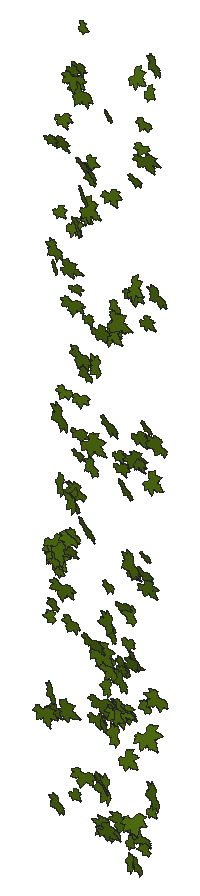
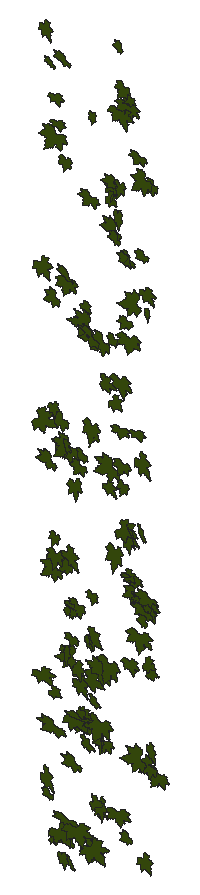
# SketchUp Ruby script. Lengths in inches.
U = 1.inch
M = Sketchup.active_model
def pt(a) = Geom::Point3d.new(a.map { |v| v * U })
def face(e, loops, mat)
  f = e.add_face(loops[0].map { |a| pt(a) })
  loops[1..].each { |l| e.add_face(l.map { |a| pt(a) }).erase! }
  f.material = f.back_material = mat if mat
  f
end
# faces: each face lists its corners as indices into pts; further lists are holes
def faces(e, pts, list, mat = nil) = list.each { |f| face(e, (f[0].is_a?(Array) ? f : [f]).map { |l| l.map { |i| pts[i] } }, mat) }
# xy, xz, yz: faces in a plane at the given z, y or x. An outline is a flat list of corners, or four numbers for a rectangle; further outlines are holes
def ring(l) = l.size == 4 ? [[l[0], l[1]], [l[2], l[1]], [l[2], l[3]], [l[0], l[3]]] : l.each_slice(2).to_a
def flat(e, list, mat, &to3) = list.each { |f| face(e, (f[0].is_a?(Array) ? f : [f]).map { |l| ring(l).map { |u, v| to3.(u, v) } }, mat) }
def xy(e, z, list, mat = nil) = flat(e, list, mat) { |x, y| [x, y, z] }
def xz(e, y, list, mat = nil) = flat(e, list, mat) { |x, z| [x, y, z] }
def yz(e, x, list, mat = nil) = flat(e, list, mat) { |y, z| [x, y, z] }
def lines(e, pts, list) = list.each { |a, b| e.add_line(pt(pts[a]), pt(pts[b])) }
# prism: a flat outline (further loops are holes) pulled along v
def prism(e, loops, v, mat = nil)
  f = face(e, loops, mat); d = Geom::Vector3d.new(v.map { |x| x * U })
  f.pushpull(f.normal.samedirection?(d) ? d.length : -d.length)
end
def box(e, o, s, mat = nil) = prism(e, [[o, [o[0] + s[0], o[1], o[2]], [o[0] + s[0], o[1] + s[1], o[2]], [o[0], o[1] + s[1], o[2]]]], [0, 0, s[2]], mat)
def at(x, y, z, deg = 0) = Geom::Transformation.translation(pt([x, y, z])) * Geom::Transformation.rotation(ORIGIN, Z_AXIS, deg.degrees)
def axes(o, x, y, z) = Geom::Transformation.new([*x, 0, *y, 0, *z, 0, *pt(o).to_a, 1])
def part(name) = M.definitions.add(name)
# library, detail: a bought-in or finely detailed component or shape, given as its bounding box
def library(name, o, s) = part(name).tap { |d| box(d.entities, o, s) }
def detail(e, o, s) = box(e.add_group.entities, o, s)
def put(e, d, t, mat = nil) = e.add_instance(d, t).tap { |i| i.material = mat if mat }
def group(e, t, mat = nil) = e.add_group.tap { |g| g.transformation = t; g.material = mat if mat }.entities
root = M.entities
M.materials.add("[Vegetation Blur 03]").color = [83, 114, 18]
c1 = part("ivy")
xy(c1.entities,0,[[0.782,0,0.786,0,0.787,0.005,0.789,0.009,0.821,0.072,0.875,0.147,1.001,0.272,1.073,0.331,1.137,0.363,1.178,0.379,1.223,0.384,1.272,0.383,1.311,0.374,1.36,0.355,1.399,0.334,1.491,0.285,1.541,0.244,1.583,0.199,1.617,0.15,1.64,0.128,1.662,0.115,1.717,0.105,1.745,0.093,1.784,0.054,1.819,0.057,1.854,0.064,1.882,0.075,1.896,0.074,1.91,0.071,1.937,0.063,1.964,0.053,1.99,0.038,2.016,0.015,2.034,0.002,2.04,0,2.038,0.003,2.036,0.007,2.033,0.038,2.036,0.068,2.045,0.1,2.055,0.116,2.064,0.123,2.077,0.129,2.088,0.129,2.106,0.132,2.118,0.13,2.179,0.132,2.207,0.133,2.225,0.133,2.242,0.138,2.22,0.162,2.207,0.186,2.206,0.213,2.212,0.236,2.228,0.262,2.247,0.274,2.298,0.283,2.355,0.294,2.37,0.296,2.376,0.295,2.377,0.3,2.377,0.303,2.385,0.329,2.411,0.37,2.426,0.392,2.449,0.407,2.511,0.426,2.561,0.444,2.619,0.466,2.589,0.469,2.561,0.476,2.501,0.5,2.449,0.516,2.424,0.523,2.401,0.535,2.377,0.556,2.372,0.568,2.36,0.575,2.268,0.586,2.225,0.592,2.207,0.599,2.194,0.61,2.143,0.65,2.13,0.664,2.122,0.682,2.123,0.7,2.13,0.719,2.148,0.75,2.17,0.781,2.195,0.807,2.221,0.828,2.284,0.874,2.291,0.88,2.288,0.887,2.276,0.9,2.267,0.916,2.265,0.933,2.273,0.967,2.292,1.002,2.313,1.03,2.334,1.054,2.348,1.067,2.358,1.074,2.363,1.076,2.362,1.081,2.35,1.094,2.347,1.11,2.35,1.143,2.359,1.18,2.385,1.254,2.415,1.324,2.448,1.393,2.45,1.4,2.446,1.398,2.44,1.394,2.427,1.383,2.402,1.36,2.376,1.339,2.345,1.324,2.305,1.309,2.282,1.303,2.273,1.306,2.245,1.294,2.212,1.287,2.187,1.291,2.163,1.301,2.142,1.316,2.134,1.327,2.124,1.325,2.09,1.292,2.053,1.259,2.014,1.234,1.973,1.215,1.954,1.21,1.931,1.208,1.909,1.212,1.893,1.22,1.879,1.233,1.872,1.248,1.867,1.281,1.864,1.319,1.821,1.258,1.773,1.197,1.726,1.141,1.698,1.121,1.679,1.116,1.666,1.117,1.647,1.122,1.632,1.129,1.62,1.141,1.617,1.154,1.617,1.219,1.621,1.254,1.623,1.268,1.623,1.281,1.618,1.314,1.606,1.346,1.603,1.375,1.607,1.403,1.603,1.467,1.599,1.499,1.605,1.525,1.614,1.552,1.629,1.577,1.635,1.589,1.629,1.587,1.618,1.582,1.596,1.566,1.581,1.556,1.568,1.552,1.557,1.55,1.545,1.553,1.531,1.562,1.522,1.572,1.504,1.591,1.486,1.611,1.474,1.631,1.457,1.666,1.455,1.684,1.457,1.698,1.452,1.715,1.444,1.728,1.424,1.754,1.419,1.772,1.423,1.786,1.434,1.819,1.444,1.848,1.446,1.855,1.44,1.861,1.43,1.867,1.386,1.904,1.349,1.948,1.326,1.973,1.31,1.995,1.288,2.048,1.284,2.153,1.287,2.254,1.284,2.255,1.282,2.253,1.278,2.247,1.274,2.237,1.266,2.216,1.226,2.125,1.208,2.076,1.184,2.033,1.155,1.984,1.135,1.942,1.111,1.899,1.083,1.861,1.053,1.85,1.059,1.83,1.061,1.809,1.056,1.79,1.049,1.767,1.04,1.749,1.018,1.733,0.994,1.726,0.942,1.734,0.95,1.6875,0.944,1.645,0.932,1.608,0.911,1.585,0.881,1.58,0.854,1.582,0.828,1.588,0.785,1.618,0.773,1.625,0.775,1.614,0.779,1.598,0.796,1.502,0.818,1.402,0.861,1.283,0.882,1.224,0.894,1.174,0.892,1.148,0.886,1.123,0.881,1.107,0.872,1.099,0.849,1.094,0.818,1.092,0.789,1.098,0.762,1.107,0.753,1.113,0.721,1.139,0.698,1.163,0.678,1.194,0.665,1.224,0.628,1.28,0.612,1.312,0.606,1.327,0.606,1.314,0.599,1.282,0.594,1.267,0.581,1.256,0.544,1.245,0.512,1.244,0.473,1.249,0.444,1.256,0.382,1.288,0.339,1.306,0.324,1.316,0.317,1.324,0.309,1.326,0.27,1.314,0.227,1.313,0.185,1.3125,0.152,1.317,0.122,1.328,0.092,1.345,0.073,1.353,0.079,1.338,0.092,1.308,0.117,1.249,0.13,1.215,0.139,1.164,0.147,1.148,0.157,1.136,0.163,1.122,0.174,1.086,0.177,1.067,0.182,1.054,0.186,1.043,0.191,1.038,0.211,1.028,0.237,1.005,0.25,0.974,0.253,0.96,0.25,0.944,0.242,0.914,0.243,0.906,0.249,0.902,0.26,0.894,0.289,0.88,0.307,0.873,0.322,0.862,0.364,0.799,0.403,0.738,0.431,0.709,0.439,0.691,0.441,0.678,0.4375,0.66,0.428,0.645,0.394,0.623,0.303,0.594,0.255,0.581,0.214,0.577,0.179,0.573,0.173,0.568,0.175,0.561,0.167,0.55,0.141,0.523,0.113,0.503,0.077,0.49,0.045,0.486,0.026,0.485,0.019,0.486,0.011,0.483,0,0.471,0.014,0.467,0.044,0.455,0.058,0.447,0.07,0.438,0.097,0.411,0.125,0.394,0.158,0.377,0.174,0.366,0.182,0.359,0.185,0.361,0.242,0.331,0.253,0.316,0.258,0.303,0.262,0.283,0.274,0.278,0.308,0.274,0.341,0.252,0.366,0.226,0.366,0.222,0.37,0.22,0.38,0.221,0.395,0.221,0.425,0.216,0.45,0.207,0.465,0.192,0.473,0.178,0.484,0.15,0.489,0.116,0.483,0.089,0.468,0.058,0.45,0.035,0.435,0.018,0.429,0.011,0.434,0.012,0.438,0.014,0.469,0.019,0.542,0.016,0.581,0.015,0.612,0.027,0.68,0.055,0.696,0.057,0.712,0.052,0.73,0.045,0.741,0.036,0.766,0.014]])
put(root,c1,axes([19.03,173.2,108.03],[0.55674,-0.05035,0.19483],[0.23814,-0.03752,-0.45478],[-0.02967,-1.24598,0.00582]),"[Vegetation Blur 03]")
put(root,c1,axes([20.39,173.2,113.54],[0.04662,-0.02211,-0.24119],[-0.29524,-0.03871,-0.03745],[0.01692,-0.61444,0.01104]),"[Vegetation Blur 03]")
put(root,c1,axes([20.4,173.2,114.15],[0.07372,0.06524,-0.26494],[-0.3259,0.04312,-0.05873],[-0.01352,-0.68368,-0.02899]),"[Vegetation Blur 03]")
put(root,c1,axes([20.1,173.2,109.72],[0.32192,-0.21102,-0.29136],[-0.33943,0.22769,-0.27574],[-0.15085,-0.96265,-0.00135]),"[Vegetation Blur 03]")
put(root,c1,axes([20.15,173.2,116.78],[0.30881,-0.07275,-0.21101],[-0.25864,0.02403,-0.25343],[-0.03462,-0.82843,0.01118]),"[Vegetation Blur 03]")
put(root,c1,axes([19.68,173.2,138.69],[0.29342,-0.08692,0.17033],[0.21238,0.06683,-0.23833],[-0.01533,-0.73794,-0.04165]),"[Vegetation Blur 03]")
put(root,c1,axes([20.23,173.2,133.52],[0.38178,-0.11889,-0.25625],[-0.31299,0.05919,-0.31491],[-0.06294,-1.01546,0.01165]),"[Vegetation Blur 03]")
put(root,c1,axes([20.39,173.2,103.86],[0.3336,-0.07994,-0.30777],[-0.37102,0.14358,-0.27372],[-0.07791,-1.02608,-0.01433]),"[Vegetation Blur 03]")
put(root,c1,axes([20.31,173.2,132.32],[0.23472,-0.16453,-0.13977],[-0.15775,0.13898,-0.20218],[-0.10411,-0.58153,-0.00877]),"[Vegetation Blur 03]")
put(root,c1,axes([19.62,173.2,117.02],[0.386,0.08915,0.27036],[0.33331,-0.03157,-0.31533],[0.02283,-1.04625,0.03255]),"[Vegetation Blur 03]")
put(root,c1,axes([19.72,173.2,108.09],[0.30498,-0.11066,0.28031],[0.34736,0.05892,-0.24807],[-0.01408,-0.94337,-0.04838]),"[Vegetation Blur 03]")
put(root,c1,axes([20.63,173.2,124.82],[0.38094,-0.16652,-0.42659],[-0.51102,0.22607,-0.31784],[-0.13644,-1.3116,-0.00062]),"[Vegetation Blur 03]")
put(root,c1,axes([20.95,173.2,120.95],[0.09708,-0.16375,-0.35064],[-0.41312,0.26056,-0.09533],[-0.14231,-0.86813,0.03753]),"[Vegetation Blur 03]")
put(root,c1,axes([19.56,173.2,116.8125],[0.58138,0.04851,0.24502],[0.30111,-0.07156,-0.47365],[0.00495,-1.34457,0.03405]),"[Vegetation Blur 03]")
put(root,c1,axes([20.21,173.2,134.86],[0.2013,0.04338,0.20783],[0.25534,-0.0094,-0.16443],[0.00948,-0.6679,0.01581]),"[Vegetation Blur 03]")
put(root,c1,axes([19.92,173.2,116.17],[0.3314,0.11464,0.31783],[0.39311,-0.13672,-0.26526],[-0.0151,-1.04335,0.06968]),"[Vegetation Blur 03]")
put(root,c1,axes([20.36,173.2,115.56],[0.07858,-0.01385,0.24493],[0.29907,-0.05144,-0.06436],[-0.02588,-0.6363,-0.00013]),"[Vegetation Blur 03]")
put(root,c1,axes([20.08,173.2,115.3],[0.62015,-0.02976,-0.03519],[-0.04222,0.07375,-0.50547],[-0.01689,-1.27709,-0.02837]),"[Vegetation Blur 03]")
put(root,c1,axes([19.98,173.2,138.72],[0.41952,-0.13561,0.24997],[0.31292,0.12999,-0.33871],[-0.01528,-1.06095,-0.07345]),"[Vegetation Blur 03]")
put(root,c1,axes([20.68,173.2,125.82],[0.33208,0.00162,-0.09351],[-0.114,-0.06757,-0.26985],[0.01145,-0.71971,0.02513]),"[Vegetation Blur 03]")
put(root,c1,axes([20.31,173.2,140.02],[0.3458,0.03513,0.16386],[0.2014,-0.03386,-0.28195],[0.00648,-0.82214,0.01861]),"[Vegetation Blur 03]")
put(root,c1,axes([21.78,173.2,120.7],[0.10352,-0.20906,-0.49577],[-0.59692,0.27823,-0.10147],[-0.15173,-1.23717,0.06096]),"[Vegetation Blur 03]")
put(root,c1,axes([20.39,173.2,108.02],[0.20638,-0.06433,0.46905],[0.57546,0.04752,-0.16762],[0.01121,-1.25569,-0.03037]),"[Vegetation Blur 03]")
put(root,c1,axes([20.77,173.2,118.04],[0.4452,0.01529,-0.01974],[-0.02317,-0.10578,-0.36101],[0.01016,-0.91136,0.04157]),"[Vegetation Blur 03]")
put(root,c1,axes([21.01,173.2,113.6875],[0.43906,-0.08807,-0.12908],[-0.15747,0.03053,-0.36003],[-0.0453,-0.95985,0.00039]),"[Vegetation Blur 03]")
put(root,c1,axes([20.74,173.2,130.61],[0.54749,0.01991,-0.01395],[-0.01748,0.04635,-0.4465],[0.00896,-1.12621,-0.01862]),"[Vegetation Blur 03]")
put(root,c1,axes([21.77,173.2,120.92],[0.16632,0.09986,-0.39596],[-0.48659,-0.03313,-0.13745],[0.03103,-1.05488,-0.03317]),"[Vegetation Blur 03]")
put(root,c1,axes([21.45,173.2,118.375],[0.23314,-0.02071,-0.23083],[-0.28282,0.0106,-0.19042],[-0.01038,-0.7542,0.00366]),"[Vegetation Blur 03]")
put(root,c1,axes([21.27,173.2,120.26],[0.37136,-0.15214,-0.22354],[-0.25515,0.22677,-0.30661],[-0.12403,-0.92207,-0.03852]),"[Vegetation Blur 03]")
put(root,c1,axes([20.87,173.2,116.9],[0.22705,-0.08947,0.23456],[0.29067,0.06726,-0.18337],[-0.00101,-0.75069,-0.04439]),"[Vegetation Blur 03]")
put(root,c1,axes([20.73,173.2,131.78],[0.15315,-0.11376,0.42127],[0.51825,0.09795,-0.12133],[0.03021,-1.10363,-0.05419]),"[Vegetation Blur 03]")
put(root,c1,axes([21.71,173.2,135.02],[0.17953,-0.09504,-0.30608],[-0.36446,0.18198,-0.15128],[-0.09974,-0.83603,0.00186]),"[Vegetation Blur 03]")
put(root,c1,axes([20.84,173.2,142.68],[0.55862,-0.01173,0.01902],[0.02312,-0.03492,-0.45573],[-0.0064,-1.15001,0.01364]),"[Vegetation Blur 03]")
put(root,c1,axes([21.03,173.2,142.86],[0.27413,-0.06194,0.16545],[0.20434,0.02916,-0.2238],[-0.01572,-0.70099,-0.02393]),"[Vegetation Blur 03]")
put(root,c1,axes([21.14,173.2,131.2],[0.28384,0.00263,0.11756],[0.14245,0.09199,-0.22943],[0.02136,-0.64851,-0.03207]),"[Vegetation Blur 03]")
put(root,c1,axes([20.98,173.2,134.24],[0.23996,0.10055,0.29847],[0.36879,-0.09254,-0.19259],[-0.01117,-0.89532,0.05342]),"[Vegetation Blur 03]")
put(root,c1,axes([21.18,173.2,104.02],[0.1988,-0.0106,0.20658],[0.25313,-0.00387,-0.16228],[-0.00466,-0.6623,-0.00236]),"[Vegetation Blur 03]")
put(root,c1,axes([21.41,173.2,122.61],[0.33381,-0.09287,0.01816],[0.028,0.08748,-0.27236],[-0.04181,-0.68286,-0.03736]),"[Vegetation Blur 03]")
put(root,c1,axes([21.28,173.2,123.66],[0.39754,-0.01789,0.09307],[0.11433,0.03939,-0.32408],[-0.00307,-0.85015,-0.01697]),"[Vegetation Blur 03]")
put(root,c1,axes([21.41,173.2,125.57],[0.37993,0.04432,0.03279],[0.04106,-0.03097,-0.31026],[0.01982,-0.78558,0.01408]),"[Vegetation Blur 03]")
put(root,c1,axes([21.32,173.2,143.3125],[0.38821,-0.11193,0.10755],[0.13579,0.05066,-0.31818],[-0.04343,-0.84212,-0.03344]),"[Vegetation Blur 03]")
put(root,c1,axes([21.48,173.2,142.46],[0.60025,-0.11632,-0.20653],[-0.25299,0.02521,-0.49198],[-0.05685,-1.34025,0.00867]),"[Vegetation Blur 03]")
put(root,c1,axes([21.42,173.2,128.3],[0.58763,-0.14391,-0.14762],[-0.17735,0.08172,-0.48275],[-0.07846,-1.26257,-0.01442]),"[Vegetation Blur 03]")
put(root,c1,axes([21.45,173.2,105.64],[0.52025,0.05923,-0.06815],[-0.08303,-0.02209,-0.42521],[0.03012,-1.08405,0.00494]),"[Vegetation Blur 03]")
put(root,c1,axes([21.62,173.2,138.35],[0.38893,-0.1332,-0.05202],[-0.05011,0.16639,-0.31658],[-0.07577,-0.79377,-0.05763]),"[Vegetation Blur 03]")
put(root,c1,axes([22.21,173.2,127.25],[0.18993,0.03098,-0.27697],[-0.33885,0.07408,-0.15347],[-0.02412,-0.79685,-0.02503]),"[Vegetation Blur 03]")
put(root,c1,axes([21.88,173.2,136.88],[0.36908,-0.2283,-0.18774],[-0.2052,0.23015,-0.31272],[-0.15204,-0.86483,-0.03366]),"[Vegetation Blur 03]")
put(root,c1,axes([21.8,173.2,145.14],[0.05613,0.01305,0.23736],[0.28926,-0.0672,-0.04498],[-0.03088,-0.6058,0.0101]),"[Vegetation Blur 03]")
put(root,c1,axes([22.53,173.2,137.81],[0.1507,0.00007,-0.27274],[-0.3307,0.10871,-0.1217],[-0.04814,-0.74651,-0.01775]),"[Vegetation Blur 03]")
put(root,c1,axes([21.8,173.2,119.22],[0.58057,-0.26082,-0.16045],[-0.16911,0.27993,-0.47915],[-0.16161,-1.22989,-0.07503]),"[Vegetation Blur 03]")
put(root,c1,axes([21.91,173.2,135.03],[0.11812,0.02268,0.27727],[0.33763,-0.09352,-0.0946],[-0.03936,-0.73423,0.02061]),"[Vegetation Blur 03]")
put(root,c1,axes([22.01,173.2,129.9],[0.26219,-0.05379,0.13773],[0.16863,-0.0189,-0.21498],[-0.02696,-0.64136,-0.00522]),"[Vegetation Blur 03]")
put(root,c1,axes([22.18,173.2,138.26],[0.41315,-0.18544,-0.14251],[-0.1576,0.18691,-0.3426],[-0.11735,-0.90388,-0.04161]),"[Vegetation Blur 03]")
put(root,c1,axes([22.55,173.2,122.61],[0.30292,-0.11557,-0.26319],[-0.32214,0.05514,-0.25077],[-0.05807,-0.90879,0.01825]),"[Vegetation Blur 03]")
put(root,c1,axes([22.18,173.2,137.93],[0.04916,0.02287,0.27993],[0.3427,0.03405,-0.04052],[0.01796,-0.71221,0.00705]),"[Vegetation Blur 03]")
put(root,c1,axes([23.12,173.2,128.08],[0.07216,-0.07343,-0.39325],[-0.48158,0.07012,-0.06092],[-0.03906,-1.00014,0.0246]),"[Vegetation Blur 03]")
put(root,c1,axes([21.84,173.2,135.25],[0.15618,0.05581,0.47785],[0.58342,-0.13447,-0.12454],[-0.05625,-1.2397,0.03502]),"[Vegetation Blur 03]")
put(root,c1,axes([21.92,173.2,113.01],[0.64437,-0.16461,0.01325],[0.02704,0.17964,-0.52482],[-0.07702,-1.31419,-0.0734]),"[Vegetation Blur 03]")
put(root,c1,axes([21.77,173.2,122.86],[0.3615,0.01419,0.44771],[0.54841,0.02846,-0.29509],[0.01534,-1.35164,-0.00151]),"[Vegetation Blur 03]")
put(root,c1,axes([22.29,173.2,108.78],[0.44477,-0.01678,0.0841],[0.10333,0.04659,-0.36253],[-0.00282,-0.93833,-0.0195]),"[Vegetation Blur 03]")
put(root,c1,axes([22.9,173.2,105.88],[0.41747,-0.18159,-0.28175],[-0.32214,0.27535,-0.34584],[-0.15229,-1.08022,-0.04079]),"[Vegetation Blur 03]")
put(root,c1,axes([23.1,173.2,109.0625],[0.30175,-0.15566,-0.18852],[-0.22184,0.13329,-0.25383],[-0.09933,-0.77056,-0.00582]),"[Vegetation Blur 03]")
put(root,c1,axes([23.59,173.2,105.9],[0.23881,-0.20013,-0.4704],[-0.57401,0.16163,-0.20491],[-0.11037,-1.27363,0.04791]),"[Vegetation Blur 03]")
put(root,c1,axes([22.29,173.2,109.81],[0.67064,-0.03297,0.06761],[0.08405,0.14038,-0.54453],[-0.00745,-1.38343,-0.05687]),"[Vegetation Blur 03]")
put(root,c1,axes([23.21,173.2,103.68],[0.46314,0.05825,-0.39602],[-0.48604,0.04033,-0.37767],[0.00535,-1.37976,-0.02776]),"[Vegetation Blur 03]")
put(root,c1,axes([22.45,173.2,129.35],[0.40049,-0.10291,0.28569],[0.35224,0.02026,-0.32774],[-0.03114,-1.09438,-0.03293]),"[Vegetation Blur 03]")
put(root,c1,axes([23.72,173.2,114.65],[0.20411,-0.06117,-0.44075],[-0.53473,0.15542,-0.16833],[-0.08116,-1.17781,0.00068]),"[Vegetation Blur 03]")
put(root,c1,axes([22.33,173.2,111.9375],[0.4004,-0.01607,0.44585],[0.54595,-0.04146,-0.32681],[-0.02086,-1.39316,0.00458]),"[Vegetation Blur 03]")
put(root,c1,axes([23.8,173.2,111.05],[0.07522,-0.13511,-0.31021],[-0.37954,0.11629,-0.06927],[-0.06884,-0.78881,0.04292]),"[Vegetation Blur 03]")
put(root,c1,axes([23.96,173.2,112.33],[0.13923,-0.07198,-0.4584],[-0.56199,0.04465,-0.11479],[-0.02951,-1.18996,0.02342]),"[Vegetation Blur 03]")
put(root,c1,axes([23.4,173.2,141.46],[0.26677,-0.13263,-0.08131],[-0.08808,0.11667,-0.22242],[-0.07951,-0.57427,-0.02641]),"[Vegetation Blur 03]")
put(root,c1,axes([23.28,173.2,116.28],[0.33233,-0.0945,-0.02615],[-0.02986,0.03657,-0.27359],[-0.04737,-0.68607,-0.01098]),"[Vegetation Blur 03]")
put(root,c1,axes([22.87,173.2,102.55],[0.26007,-0.08689,0.38147],[0.46915,0.07766,-0.21026],[0.0126,-1.09796,-0.04506]),"[Vegetation Blur 03]")
put(root,c1,axes([23.11,173.2,125.13],[0.58072,-0.2362,-0.06513],[-0.0644,0.17074,-0.47989],[-0.12408,-1.1941,-0.05574]),"[Vegetation Blur 03]")
put(root,c1,axes([23.84,173.2,114.08],[0.25432,-0.19046,-0.24423],[-0.28944,0.16036,-0.22043],[-0.11975,-0.79207,0.0141]),"[Vegetation Blur 03]")
put(root,c1,axes([23.08,173.2,136.9],[0.40459,0.02303,0.19859],[0.2435,-0.01333,-0.3302],[0.00625,-0.97145,0.00924]),"[Vegetation Blur 03]")
put(root,c1,axes([24.27,173.2,108.75],[0.10121,-0.15146,-0.36108],[-0.44341,0.10659,-0.08981],[-0.06746,-0.92784,0.04863]),"[Vegetation Blur 03]")
put(root,c1,axes([23.98,173.2,131.5],[0.20022,-0.05357,-0.19807],[-0.24233,0.03356,-0.1646],[-0.02917,-0.64656,0.00787]),"[Vegetation Blur 03]")
put(root,c1,axes([24.29,173.2,110.2],[0.11196,0.05174,-0.31654],[-0.38834,-0.01941,-0.09199],[0.01605,-0.83049,-0.01757]),"[Vegetation Blur 03]")
put(root,c1,axes([23.05,173.2,129.24],[0.28098,0.0713,0.44477],[0.5442,-0.14112,-0.22543],[-0.04527,-1.25382,0.05067]),"[Vegetation Blur 03]")
put(root,c1,axes([23.58,173.2,108.81],[0.09158,0.04301,0.34718],[0.42504,-0.06647,-0.07338],[-0.02723,-0.89296,0.02219]),"[Vegetation Blur 03]")
put(root,c1,axes([24.23,173.2,111.93],[0.35185,-0.14327,-0.37157],[-0.44566,0.19161,-0.29272],[-0.11623,-1.16844,-0.00244]),"[Vegetation Blur 03]")
put(root,c1,axes([24.09,173.2,110.13],[0.45581,0.11699,-0.31525],[-0.38742,-0.0162,-0.37405],[0.04848,-1.22937,-0.02507]),"[Vegetation Blur 03]")
put(root,c1,axes([23.82,173.2,104.16],[0.58678,0.063,-0.19417],[-0.23912,0.05083,-0.47872],[0.01906,-1.30195,-0.02809]),"[Vegetation Blur 03]")
put(root,c1,axes([23.33,173.2,109.53],[0.59488,0.11123,0.16598],[0.20655,-0.0688,-0.48585],[0.04022,-1.29188,0.04016]),"[Vegetation Blur 03]")
put(root,c1,axes([23.51,173.2,129.59],[0.09221,0.01276,0.54145],[0.66339,-0.02223,-0.07517],[-0.00985,-1.37816,0.00623]),"[Vegetation Blur 03]")
put(root,c1,axes([23.8,173.2,123.17],[0.25,-0.03131,0.17773],[0.21716,-0.03407,-0.2044],[-0.02234,-0.68141,0.00205]),"[Vegetation Blur 03]")
put(root,c1,axes([24.24,173.2,112.5625],[0.39633,-0.13888,-0.234],[-0.27566,0.17367,-0.32719],[-0.1038,-0.99151,-0.02453]),"[Vegetation Blur 03]")
put(root,c1,axes([23.82,173.2,122.63],[0.3534,-0.02851,0.14206],[0.17452,0.03242,-0.28817],[-0.00545,-0.81,-0.01653]),"[Vegetation Blur 03]")
put(root,c1,axes([24.27,173.2,122.03],[0.4235,-0.13743,-0.21645],[-0.24668,0.24247,-0.3457],[-0.1181,-0.99928,-0.05411]),"[Vegetation Blur 03]")
put(root,c1,axes([24.04,173.2,111.86],[0.26031,-0.0805,0.12545],[0.1556,0.01165,-0.21388],[-0.03078,-0.62197,-0.02024]),"[Vegetation Blur 03]")
put(root,c1,axes([23.91,173.2,115.28],[0.41549,-0.08208,0.11963],[0.15106,0.12998,-0.33542],[-0.01613,-0.89729,-0.05953]),"[Vegetation Blur 03]")
put(root,c1,axes([25.2,173.2,115.46],[0.08632,-0.07212,-0.36138],[-0.4424,0.06914,-0.07256],[-0.03977,-0.92577,0.02273]),"[Vegetation Blur 03]")
put(root,c1,axes([24.88,173.2,118.4375],[0.39881,-0.16855,-0.40776],[-0.49292,0.16963,-0.33214],[-0.11562,-1.30452,0.00949]),"[Vegetation Blur 03]")
put(root,c1,axes([25.11,173.2,102.12],[0.10497,-0.16799,-0.28426],[-0.34085,0.17977,-0.10055],[-0.10859,-0.72666,0.04084]),"[Vegetation Blur 03]")
put(root,c1,axes([24.375,173.2,113.5625],[0.3425,-0.04443,0.04433],[0.05384,-0.01893,-0.28004],[-0.02276,-0.71335,0.00467]),"[Vegetation Blur 03]")
put(root,c1,axes([24.08,173.2,106.75],[0.24435,0.09355,0.35761],[0.44053,-0.04867,-0.19849],[0.00137,-1.03125,0.04181]),"[Vegetation Blur 03]")
put(root,c1,axes([24.6,173.2,102.54],[0.09713,0.02395,0.23937],[0.28996,-0.10667,-0.07669],[-0.04564,-0.62678,0.0222]),"[Vegetation Blur 03]")
put(root,c1,axes([24.41,173.2,132.24],[0.48068,0.01776,0.03152],[0.03794,0.06838,-0.39147],[0.01124,-0.98997,-0.02647]),"[Vegetation Blur 03]")
put(root,c1,axes([24.94,173.2,113.05],[0.36602,-0.17334,-0.17958],[-0.2031,0.19186,-0.30487],[-0.11941,-0.85763,-0.0319]),"[Vegetation Blur 03]")
put(root,c1,axes([24.77,173.2,138.55],[0.37054,-0.08411,-0.02834],[-0.02969,0.09383,-0.30232],[-0.04467,-0.76008,-0.03419]),"[Vegetation Blur 03]")
put(root,c1,axes([24.32,173.2,103.84],[0.46596,0.12424,0.22352],[0.28037,-0.18097,-0.37349],[0.00652,-1.09739,0.0869]),"[Vegetation Blur 03]")
put(root,c1,axes([24.65,173.2,117.06],[0.25004,-0.05522,0.19659],[0.24228,0.07618,-0.20189],[0.00655,-0.71038,-0.03693]),"[Vegetation Blur 03]")
put(root,c1,axes([25.15,173.2,103.81],[0.43018,0.03461,-0.33433],[-0.40999,0.03807,-0.35076],[-0.00059,-1.2218,-0.0204]),"[Vegetation Blur 03]")
put(root,c1,axes([24.58,173.2,112.03],[0.13975,-0.17275,0.35559],[0.44281,0.11446,-0.10717],[0.0284,-0.9346,-0.07885]),"[Vegetation Blur 03]")
put(root,c1,axes([24.64,173.2,131.97],[0.08788,0.15958,0.41108],[0.50211,-0.20702,-0.05886],[-0.08717,-1.03158,0.0754]),"[Vegetation Blur 03]")
put(root,c1,axes([24.24,173.2,123.21],[0.49372,-0.08066,0.3359],[0.41334,0.06825,-0.4021],[-0.00879,-1.32093,-0.04129]),"[Vegetation Blur 03]")
put(root,c1,axes([25.14,173.2,102.14],[0.34936,-0.1754,-0.17065],[-0.20005,0.12722,-0.29335],[-0.10473,-0.82812,-0.00892]),"[Vegetation Blur 03]")
put(root,c1,axes([24.96,173.2,123.82],[0.46927,-0.11869,-0.14311],[-0.17217,0.07416,-0.3857],[-0.06659,-1.02821,-0.0113]),"[Vegetation Blur 03]")
put(root,c1,axes([24.74,173.2,143.34],[0.1221,0.15901,0.36769],[0.45566,-0.11863,-0.09271],[-0.03634,-0.95319,0.07288]),"[Vegetation Blur 03]")
put(root,c1,axes([25.27,173.2,140.4],[0.32282,0.01218,-0.05233],[-0.06347,-0.05325,-0.26277],[0.01083,-0.67519,0.01978]),"[Vegetation Blur 03]")
put(root,c1,axes([24.86,173.2,124.54],[0.35919,-0.07581,0.24051],[0.29623,0.02355,-0.29351],[-0.02119,-0.9558,-0.02631]),"[Vegetation Blur 03]")
put(root,c1,axes([25.44,173.2,141.8],[0.32239,-0.01176,-0.10948],[-0.13423,-0.01041,-0.2631],[-0.00333,-0.71849,0.00561]),"[Vegetation Blur 03]")
put(root,c1,axes([25.96,173.2,103.01],[0.06839,0.01536,-0.24268],[-0.29667,-0.04173,-0.0561],[0.02144,-0.62648,-0.00221]),"[Vegetation Blur 03]")
put(root,c1,axes([25.86,173.2,110.71],[0.15181,-0.00524,-0.23084],[-0.28286,-0.00517,-0.12389],[0.00101,-0.66057,0.0028]),"[Vegetation Blur 03]")
put(root,c1,axes([25.62,173.2,125.6],[0.28037,-0.06157,-0.15463],[-0.18018,0.15229,-0.22714],[-0.06579,-0.67947,-0.0369]),"[Vegetation Blur 03]")
put(root,c1,axes([25.22,173.2,117.7],[0.47998,-0.11829,-0.01678],[-0.01365,0.11877,-0.39191],[-0.0595,-0.98146,-0.0454]),"[Vegetation Blur 03]")
put(root,c1,axes([25.45,173.2,118.55],[0.3065,-0.10801,0.00878],[0.01921,0.10156,-0.25024],[-0.05001,-0.62289,-0.04232]),"[Vegetation Blur 03]")
put(root,c1,axes([24.9,173.2,139.53],[0.56255,-0.01811,0.20546],[0.25121,0.13405,-0.45628],[0.01862,-1.26114,-0.05145]),"[Vegetation Blur 03]")
put(root,c1,axes([24.96,173.2,108.34],[0.39393,0.1891,0.39235],[0.48905,-0.10099,-0.3194],[0.01969,-1.27498,0.08349]),"[Vegetation Blur 03]")
put(root,c1,axes([25.39,173.2,130.7],[0.23197,-0.0436,0.29061],[0.3566,0.00644,-0.18945],[-0.00894,-0.8745,-0.01588]),"[Vegetation Blur 03]")
put(root,c1,axes([26.34,173.2,106.44],[0.28462,-0.17247,-0.45638],[-0.54186,0.28495,-0.24203],[-0.16158,-1.25936,0.00774]),"[Vegetation Blur 03]")
put(root,c1,axes([25.2,173.2,116.58],[0.39343,-0.07208,0.30532],[0.37571,0.06003,-0.32024],[-0.0052,-1.11557,-0.03696]),"[Vegetation Blur 03]")
put(root,c1,axes([25.69,173.2,142.95],[0.0888,0.09674,0.25308],[0.31076,-0.1168,-0.0656],[-0.0424,-0.6534,0.0492]),"[Vegetation Blur 03]")
put(root,c1,axes([26.64,173.2,125.1],[0.14596,0.116,-0.44941],[-0.55223,-0.05004,-0.12149],[0.03805,-1.17121,-0.03932]),"[Vegetation Blur 03]")
put(root,c1,axes([26.2,173.2,145.45],[0.35368,-0.15187,-0.29343],[-0.34945,0.17479,-0.29479],[-0.11221,-1.02299,-0.00681]),"[Vegetation Blur 03]")
put(root,c1,axes([25.79,173.2,104.72],[0.17985,0.03398,0.21034],[0.25744,-0.07475,-0.14472],[-0.02044,-0.64238,0.02797]),"[Vegetation Blur 03]")
put(root,c1,axes([26.29,173.2,133.11],[0.38374,-0.03816,-0.34105],[-0.41282,0.15382,-0.31209],[-0.06752,-1.15732,-0.03024]),"[Vegetation Blur 03]")
put(root,c1,axes([25.59,173.2,121.98],[0.16307,0.08475,0.41488],[0.5096,-0.07153,-0.13111],[-0.02064,-1.09626,0.04063]),"[Vegetation Blur 03]")
put(root,c1,axes([26.22,173.2,111.56],[0.42678,-0.01115,-0.26433],[-0.32354,-0.0687,-0.34749],[0.01587,-1.10035,0.02437]),"[Vegetation Blur 03]")
